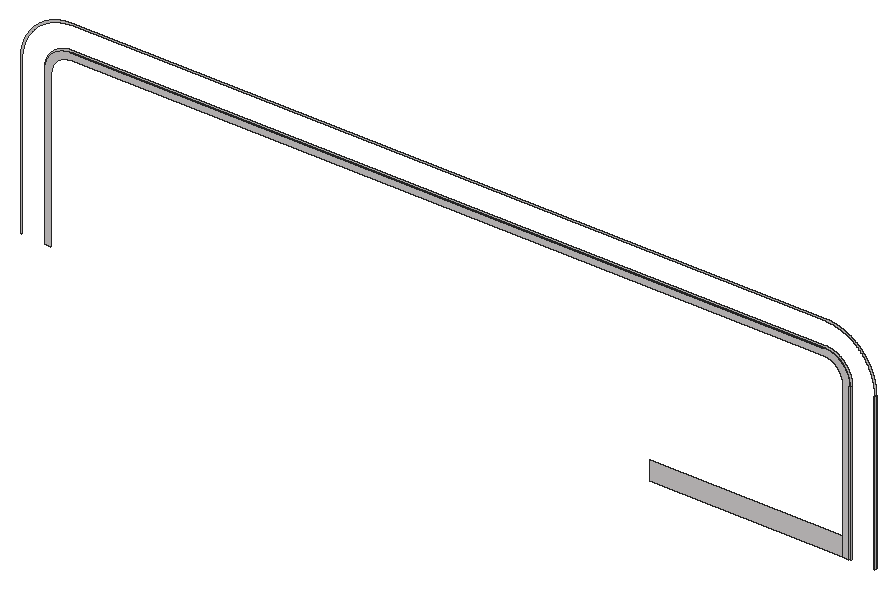
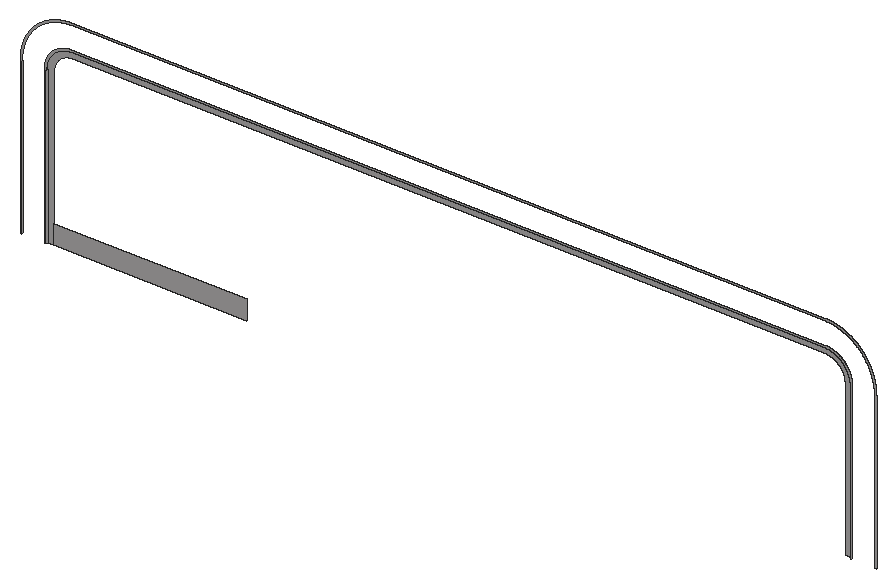
# SketchUp Ruby script. Lengths in inches.
U = 1.inch
M = Sketchup.active_model
def pt(a) = Geom::Point3d.new(a.map { |v| v * U })
def face(e, loops, mat)
  f = e.add_face(loops[0].map { |a| pt(a) })
  loops[1..].each { |l| e.add_face(l.map { |a| pt(a) }).erase! }
  f.material = f.back_material = mat if mat
  f
end
# faces: each face lists its corners as indices into pts; further lists are holes
def faces(e, pts, list, mat = nil) = list.each { |f| face(e, (f[0].is_a?(Array) ? f : [f]).map { |l| l.map { |i| pts[i] } }, mat) }
# xy, xz, yz: faces in a plane at the given z, y or x. An outline is a flat list of corners, or four numbers for a rectangle; further outlines are holes
def ring(l) = l.size == 4 ? [[l[0], l[1]], [l[2], l[1]], [l[2], l[3]], [l[0], l[3]]] : l.each_slice(2).to_a
def flat(e, list, mat, &to3) = list.each { |f| face(e, (f[0].is_a?(Array) ? f : [f]).map { |l| ring(l).map { |u, v| to3.(u, v) } }, mat) }
def xy(e, z, list, mat = nil) = flat(e, list, mat) { |x, y| [x, y, z] }
def xz(e, y, list, mat = nil) = flat(e, list, mat) { |x, z| [x, y, z] }
def yz(e, x, list, mat = nil) = flat(e, list, mat) { |y, z| [x, y, z] }
def lines(e, pts, list) = list.each { |a, b| e.add_line(pt(pts[a]), pt(pts[b])) }
# prism: a flat outline (further loops are holes) pulled along v
def prism(e, loops, v, mat = nil)
  f = face(e, loops, mat); d = Geom::Vector3d.new(v.map { |x| x * U })
  f.pushpull(f.normal.samedirection?(d) ? d.length : -d.length)
end
def box(e, o, s, mat = nil) = prism(e, [[o, [o[0] + s[0], o[1], o[2]], [o[0] + s[0], o[1] + s[1], o[2]], [o[0], o[1] + s[1], o[2]]]], [0, 0, s[2]], mat)
def at(x, y, z, deg = 0) = Geom::Transformation.translation(pt([x, y, z])) * Geom::Transformation.rotation(ORIGIN, Z_AXIS, deg.degrees)
def axes(o, x, y, z) = Geom::Transformation.new([*x, 0, *y, 0, *z, 0, *pt(o).to_a, 1])
def part(name) = M.definitions.add(name)
# library, detail: a bought-in or finely detailed component or shape, given as its bounding box
def library(name, o, s) = part(name).tap { |d| box(d.entities, o, s) }
def detail(e, o, s) = box(e.add_group.entities, o, s)
def put(e, d, t, mat = nil) = e.add_instance(d, t).tap { |i| i.material = mat if mat }
def group(e, t, mat = nil) = e.add_group.tap { |g| g.transformation = t; g.material = mat if mat }.entities
root = M.entities
M.materials.add("[Quartz Light Brown]").color = [215, 212, 212]
xz(root,38,[[20,-12,24,-12,24,84.28,24.01,84.375,24.01,84.57,24.02,84.66,24.02,84.75,24.03,84.85,24.04,84.94,24.04,85.04,24.05,85.13,24.0625,85.22,24.07,85.32,24.09,85.5,24.11,85.6,24.13,85.78,24.15,85.88,24.16,85.97,24.18,86.0625,24.2,86.16,24.21,86.25,24.25,86.43,24.27,86.53,24.35,86.89,24.38,86.98,24.4,87.08,24.43,87.17,24.45,87.26,24.48,87.35,24.5,87.4375,24.53,87.53,24.68,87.98,24.71,88.06,24.77,88.24,24.81,88.33,24.84,88.42,24.88,88.5,24.91,88.59,24.99,88.77,25.02,88.85,25.0625,88.9375,25.1,89.02,25.14,89.11,25.18,89.19,25.22,89.28,25.27,89.36,25.31,89.45,25.35,89.53,25.39,89.62,25.4375,89.7,25.48,89.78,25.53,89.86,25.58,89.95,25.67,90.11,25.72,90.1875,25.77,90.27,26.02,90.67,26.08,90.75,26.13,90.82,26.18,90.9,26.24,90.98,26.29,91.05,26.35,91.13,26.4,91.21,26.52,91.35,26.58,91.43,26.63,91.5,26.69,91.58,26.75,91.65,26.9375,91.86,27,91.9375,27.0625,92.01,27.1875,92.15,27.25,92.21,27.32,92.28,27.38,92.35,27.45,92.42,27.51,92.49,27.58,92.55,27.65,92.62,27.72,92.68,27.79,92.75,27.85,92.8125,27.99,92.9375,28.0625,93,28.14,93.0625,28.35,93.25,28.42,93.31,28.5,93.37,28.57,93.42,28.65,93.48,28.79,93.6,28.87,93.65,28.95,93.71,29.02,93.76,29.1,93.82,29.18,93.87,29.25,93.92,29.33,93.98,29.73,94.23,29.8125,94.28,29.89,94.33,30.05,94.42,30.14,94.47,30.22,94.52,30.3,94.5625,30.38,94.61,30.47,94.65,30.55,94.69,30.64,94.73,30.72,94.78,30.81,94.82,30.89,94.86,30.98,94.9,31.0625,94.9375,31.15,94.98,31.23,95.01,31.41,95.09,31.5,95.12,31.58,95.16,31.67,95.19,31.76,95.23,31.94,95.29,32.02,95.32,32.47,95.47,32.5625,95.5,32.65,95.52,32.74,95.55,32.83,95.57,32.92,95.6,33.02,95.62,33.11,95.65,33.47,95.73,33.57,95.75,33.75,95.79,33.84,95.8,33.9375,95.82,34.03,95.84,34.12,95.85,34.22,95.87,34.4,95.89,34.5,95.91,34.68,95.93,34.78,95.9375,34.87,95.95,34.96,95.96,35.06,95.96,35.15,95.97,35.25,95.98,35.34,95.98,35.43,95.99,35.625,95.99,35.72,96,504.28,96,504.375,95.99,504.57,95.99,504.66,95.98,504.75,95.98,504.85,95.97,504.94,95.96,505.04,95.96,505.13,95.95,505.22,95.9375,505.32,95.93,505.5,95.91,505.6,95.89,505.78,95.87,505.88,95.85,505.97,95.84,506.0625,95.82,506.16,95.8,506.25,95.79,506.43,95.75,506.53,95.73,506.89,95.65,506.98,95.62,507.08,95.6,507.17,95.57,507.26,95.55,507.35,95.52,507.4375,95.5,507.53,95.47,507.98,95.32,508.06,95.29,508.24,95.23,508.33,95.19,508.42,95.16,508.5,95.12,508.59,95.09,508.77,95.01,508.85,94.98,508.9375,94.9375,509.02,94.9,509.11,94.86,509.19,94.82,509.28,94.78,509.36,94.73,509.45,94.69,509.53,94.65,509.62,94.61,509.7,94.5625,509.78,94.52,509.86,94.47,509.95,94.42,510.11,94.33,510.1875,94.28,510.27,94.23,510.67,93.98,510.75,93.92,510.82,93.87,510.9,93.82,510.98,93.76,511.05,93.71,511.13,93.65,511.21,93.6,511.35,93.48,511.43,93.42,511.5,93.37,511.58,93.31,511.65,93.25,511.86,93.0625,511.9375,93,512.01,92.9375,512.15,92.8125,512.21,92.75,512.28,92.68,512.35,92.62,512.42,92.55,512.49,92.49,512.55,92.42,512.62,92.35,512.68,92.28,512.75,92.21,512.8125,92.15,512.9375,92.01,513,91.9375,513.0625,91.86,513.25,91.65,513.31,91.58,513.37,91.5,513.42,91.43,513.48,91.35,513.6,91.21,513.65,91.13,513.71,91.05,513.76,90.98,513.82,90.9,513.87,90.82,513.92,90.75,513.98,90.67,514.23,90.27,514.28,90.1875,514.33,90.11,514.42,89.95,514.47,89.86,514.52,89.78,514.5625,89.7,514.61,89.62,514.65,89.53,514.69,89.45,514.73,89.36,514.78,89.28,514.82,89.19,514.86,89.11,514.9,89.02,514.9375,88.9375,514.98,88.85,515.01,88.77,515.09,88.59,515.12,88.5,515.16,88.42,515.19,88.33,515.23,88.24,515.29,88.06,515.32,87.98,515.47,87.53,515.5,87.4375,515.52,87.35,515.55,87.26,515.57,87.17,515.6,87.08,515.62,86.98,515.65,86.89,515.73,86.53,515.75,86.43,515.79,86.25,515.8,86.16,515.82,86.0625,515.84,85.97,515.85,85.88,515.87,85.78,515.89,85.6,515.91,85.5,515.93,85.32,515.9375,85.22,515.95,85.13,515.96,85.04,515.96,84.94,515.97,84.85,515.98,84.75,515.98,84.66,515.99,84.57,515.99,84.375,516,84.28,516,-12,520,-12,520,84.375,519.99,84.5,519.99,84.63,519.98,84.75,519.98,84.88,519.97,85,519.95,85.26,519.94,85.38,519.93,85.51,519.92,85.63,519.9,85.76,519.89,85.88,519.875,86.01,519.86,86.13,519.84,86.25,519.82,86.38,519.8,86.5,519.72,87,519.69,87.12,519.67,87.24,519.64,87.37,519.61,87.49,519.59,87.61,519.56,87.74,519.47,88.1,519.43,88.22,519.4,88.34,519.36,88.46,519.33,88.58,519.29,88.7,519.26,88.82,519.22,88.94,519.18,89.0625,519.14,89.18,519.1,89.3,519.05,89.42,518.97,89.66,518.92,89.77,518.83,90.01,518.78,90.12,518.73,90.24,518.68,90.35,518.63,90.47,518.58,90.58,518.53,90.7,518.48,90.8125,518.42,90.93,518.37,91.04,518.3125,91.15,518.26,91.26,518.14,91.49,517.84,92.04,517.77,92.14,517.71,92.25,517.64,92.36,517.58,92.47,517.51,92.57,517.44,92.68,517.37,92.78,517.3,92.89,517.23,92.99,517.16,93.1,517.02,93.3,516.94,93.4,516.87,93.51,516.79,93.61,516.72,93.71,516.56,93.91,516.49,94,516.25,94.3,516.17,94.39,516.08,94.49,515.92,94.67,515.83,94.77,515.75,94.86,515.66,94.95,515.58,95.04,515.4,95.22,515.3125,95.3125,515.22,95.4,515.04,95.58,514.95,95.66,514.86,95.75,514.77,95.83,514.67,95.92,514.49,96.08,514.39,96.17,514.3,96.25,514,96.49,513.91,96.56,513.71,96.72,513.61,96.79,513.51,96.87,513.4,96.94,513.3,97.02,513.1,97.16,512.99,97.23,512.89,97.3,512.78,97.37,512.68,97.44,512.57,97.51,512.47,97.58,512.36,97.64,512.25,97.71,512.14,97.77,512.04,97.84,511.49,98.14,511.26,98.26,511.15,98.3125,511.04,98.37,510.93,98.42,510.8125,98.48,510.7,98.53,510.58,98.58,510.47,98.63,510.35,98.68,510.24,98.73,510.12,98.78,510.01,98.83,509.77,98.92,509.66,98.97,509.42,99.05,509.3,99.1,509.18,99.14,509.0625,99.18,508.94,99.22,508.82,99.26,508.7,99.29,508.58,99.33,508.46,99.36,508.34,99.4,508.22,99.43,508.1,99.47,507.74,99.56,507.61,99.59,507.49,99.61,507.37,99.64,507.24,99.67,507.12,99.69,507,99.72,506.5,99.8,506.38,99.82,506.25,99.84,506.13,99.86,506.01,99.875,505.88,99.89,505.76,99.9,505.63,99.92,505.51,99.93,505.38,99.94,505.26,99.95,505,99.97,504.88,99.98,504.75,99.98,504.63,99.99,504.5,99.99,504.375,100,35.625,100,35.5,99.99,35.37,99.99,35.25,99.98,35.12,99.98,35,99.97,34.74,99.95,34.62,99.94,34.49,99.93,34.37,99.92,34.24,99.9,34.12,99.89,33.99,99.875,33.87,99.86,33.75,99.84,33.62,99.82,33.5,99.8,33,99.72,32.88,99.69,32.76,99.67,32.63,99.64,32.51,99.61,32.39,99.59,32.26,99.56,31.9,99.47,31.78,99.43,31.66,99.4,31.54,99.36,31.42,99.33,31.3,99.29,31.18,99.26,31.06,99.22,30.9375,99.18,30.82,99.14,30.7,99.1,30.58,99.05,30.34,98.97,30.23,98.92,29.99,98.83,29.88,98.78,29.76,98.73,29.65,98.68,29.53,98.63,29.42,98.58,29.3,98.53,29.1875,98.48,29.07,98.42,28.96,98.37,28.85,98.3125,28.74,98.26,28.51,98.14,27.96,97.84,27.86,97.77,27.75,97.71,27.64,97.64,27.53,97.58,27.43,97.51,27.32,97.44,27.22,97.37,27.11,97.3,27.01,97.23,26.9,97.16,26.7,97.02,26.6,96.94,26.49,96.87,26.39,96.79,26.29,96.72,26.09,96.56,26,96.49,25.7,96.25,25.61,96.17,25.51,96.08,25.33,95.92,25.23,95.83,25.14,95.75,25.05,95.66,24.96,95.58,24.78,95.4,24.6875,95.3125,24.6,95.22,24.42,95.04,24.34,94.95,24.25,94.86,24.17,94.77,24.08,94.67,23.92,94.49,23.83,94.39,23.75,94.3,23.51,94,23.44,93.91,23.28,93.71,23.21,93.61,23.13,93.51,23.06,93.4,22.98,93.3,22.84,93.1,22.77,92.99,22.7,92.89,22.63,92.78,22.56,92.68,22.49,92.57,22.42,92.47,22.36,92.36,22.29,92.25,22.23,92.14,22.16,92.04,21.86,91.49,21.74,91.26,21.6875,91.15,21.63,91.04,21.58,90.93,21.52,90.8125,21.47,90.7,21.42,90.58,21.37,90.47,21.32,90.35,21.27,90.24,21.22,90.12,21.17,90.01,21.08,89.77,21.03,89.66,20.95,89.42,20.9,89.3,20.86,89.18,20.82,89.0625,20.78,88.94,20.74,88.82,20.71,88.7,20.67,88.58,20.64,88.46,20.6,88.34,20.57,88.22,20.53,88.1,20.44,87.74,20.41,87.61,20.39,87.49,20.36,87.37,20.33,87.24,20.31,87.12,20.28,87,20.2,86.5,20.18,86.38,20.16,86.25,20.14,86.13,20.125,86.01,20.11,85.88,20.1,85.76,20.08,85.63,20.07,85.51,20.06,85.38,20.05,85.26,20.03,85,20.02,84.88,20.02,84.75,20.01,84.63,20.01,84.5,20,84.375],[396,-12,516,0]],"[Quartz Light Brown]")
xz(root,39,[[4,-12,5,-12,5,84.49,5.02,84.97,5.02,85.22,5.03,85.46,5.05,85.7,5.0625,85.95,5.08,86.1875,5.1,86.43,5.12,86.67,5.14,86.92,5.16,87.16,5.1875,87.4,5.21,87.64,5.24,87.89,5.28,88.125,5.31,88.37,5.34,88.61,5.5,89.57,5.6,90.05,5.64,90.29,5.69,90.52,5.75,90.76,5.8,91,5.86,91.24,5.91,91.47,5.97,91.71,6.04,91.94,6.1,92.18,6.16,92.41,6.23,92.65,6.3,92.88,6.37,93.12,6.44,93.35,6.52,93.58,6.59,93.8125,6.67,94.04,6.83,94.5,6.92,94.73,7,94.96,7.09,95.19,7.18,95.41,7.27,95.64,7.36,95.86,7.45,96.09,7.55,96.3125,7.65,96.53,7.75,96.76,8.05,97.42,8.27,97.86,8.38,98.07,8.6,98.51,8.72,98.72,8.83,98.93,8.95,99.15,9.19,99.57,9.32,99.78,9.44,99.99,9.57,100.2,9.7,100.4,9.96,100.82,10.22,101.22,10.36,101.42,10.64,101.83,10.78,102.02,10.92,102.22,11.0625,102.42,11.21,102.61,11.36,102.81,12.11,103.76,12.27,103.95,12.43,104.13,12.59,104.32,13.07,104.86,13.24,105.04,13.4,105.22,13.57,105.4,13.74,105.57,13.91,105.75,14.25,106.09,14.43,106.26,14.6,106.43,14.78,106.6,14.96,106.76,15.14,106.93,15.68,107.41,15.87,107.57,16.05,107.73,16.24,107.89,17.19,108.64,17.39,108.79,17.58,108.9375,17.78,109.08,17.98,109.22,18.17,109.36,18.58,109.64,18.78,109.78,19.18,110.04,19.6,110.3,19.8,110.43,20.01,110.56,20.22,110.68,20.43,110.81,20.85,111.05,21.07,111.17,21.28,111.28,21.49,111.4,21.93,111.62,22.14,111.73,22.58,111.95,23.24,112.25,23.47,112.35,23.6875,112.45,23.91,112.55,24.14,112.64,24.36,112.73,24.59,112.82,24.81,112.91,25.04,113,25.27,113.08,25.5,113.17,25.96,113.33,26.1875,113.41,26.42,113.48,26.65,113.56,26.88,113.63,27.12,113.7,27.35,113.77,27.59,113.84,27.82,113.9,28.06,113.96,28.29,114.03,28.53,114.09,28.76,114.14,29,114.2,29.24,114.25,29.48,114.31,29.71,114.36,29.95,114.4,30.43,114.5,31.39,114.66,31.63,114.69,31.875,114.72,32.11,114.76,32.36,114.79,32.6,114.8125,32.84,114.84,33.08,114.86,33.33,114.88,33.57,114.9,33.8125,114.92,34.05,114.9375,34.3,114.95,34.54,114.97,34.78,114.98,35.03,114.98,35.51,115,504.49,115,504.97,114.98,505.22,114.98,505.46,114.97,505.7,114.95,505.95,114.9375,506.1875,114.92,506.43,114.9,506.67,114.88,506.92,114.86,507.16,114.84,507.4,114.8125,507.64,114.79,507.89,114.76,508.125,114.72,508.37,114.69,508.61,114.66,509.57,114.5,510.05,114.4,510.29,114.36,510.52,114.31,510.76,114.25,511,114.2,511.24,114.14,511.47,114.09,511.71,114.03,511.94,113.96,512.18,113.9,512.41,113.84,512.65,113.77,512.88,113.7,513.12,113.63,513.35,113.56,513.58,113.48,513.8125,113.41,514.04,113.33,514.5,113.17,514.73,113.08,514.96,113,515.19,112.91,515.41,112.82,515.64,112.73,515.86,112.64,516.09,112.55,516.3125,112.45,516.53,112.35,516.76,112.25,517.42,111.95,517.86,111.73,518.07,111.62,518.51,111.4,518.72,111.28,518.93,111.17,519.15,111.05,519.57,110.81,519.78,110.68,519.99,110.56,520.2,110.43,520.4,110.3,520.82,110.04,521.22,109.78,521.42,109.64,521.83,109.36,522.02,109.22,522.22,109.08,522.42,108.9375,522.61,108.79,522.81,108.64,523.76,107.89,523.95,107.73,524.13,107.57,524.32,107.41,524.86,106.93,525.04,106.76,525.22,106.6,525.4,106.43,525.57,106.26,525.75,106.09,526.09,105.75,526.26,105.57,526.43,105.4,526.6,105.22,526.76,105.04,526.93,104.86,527.41,104.32,527.57,104.13,527.73,103.95,527.89,103.76,528.64,102.81,528.79,102.61,528.9375,102.42,529.08,102.22,529.22,102.02,529.36,101.83,529.64,101.42,529.78,101.22,530.04,100.82,530.3,100.4,530.43,100.2,530.56,99.99,530.68,99.78,530.81,99.57,531.05,99.15,531.17,98.93,531.28,98.72,531.4,98.51,531.62,98.07,531.73,97.86,531.95,97.42,532.25,96.76,532.35,96.53,532.45,96.3125,532.55,96.09,532.64,95.86,532.73,95.64,532.82,95.41,532.91,95.19,533,94.96,533.08,94.73,533.17,94.5,533.33,94.04,533.41,93.8125,533.48,93.58,533.56,93.35,533.63,93.12,533.7,92.88,533.77,92.65,533.84,92.41,533.9,92.18,533.96,91.94,534.03,91.71,534.09,91.47,534.14,91.24,534.2,91,534.25,90.76,534.31,90.52,534.36,90.29,534.4,90.05,534.5,89.57,534.66,88.61,534.69,88.37,534.72,88.125,534.76,87.89,534.79,87.64,534.8125,87.4,534.84,87.16,534.86,86.92,534.88,86.67,534.9,86.43,534.92,86.1875,534.9375,85.95,534.95,85.7,534.97,85.46,534.98,85.22,534.98,84.97,535,84.49,535,-12,536,-12,536,84.5,535.99,84.75,535.98,85.01,535.98,85.26,535.96,85.51,535.95,85.76,535.9375,86.01,535.92,86.26,535.86,87.01,535.83,87.26,535.81,87.51,535.72,88.26,535.64,88.76,535.61,89.01,535.57,89.25,535.52,89.5,535.48,89.75,535.43,90,535.39,90.24,535.34,90.49,535.28,90.74,535.23,90.98,535.17,91.23,535.12,91.47,535.06,91.71,534.99,91.96,534.87,92.44,534.8,92.6875,534.73,92.93,534.59,93.41,534.43,93.89,534.36,94.13,534.27,94.37,534.19,94.6,534.11,94.84,534.02,95.08,533.93,95.3125,533.84,95.55,533.66,96.01,533.5625,96.25,533.47,96.48,533.37,96.71,533.27,96.9375,533.16,97.17,533.0625,97.4,532.95,97.625,532.85,97.85,532.74,98.08,532.625,98.3,532.4,98.75,532.28,98.97,532.16,99.2,531.92,99.64,531.8,99.85,531.41,100.51,531.15,100.93,531.02,101.15,530.88,101.36,530.75,101.57,530.47,101.99,530.32,102.19,530.04,102.61,529.59,103.21,529.4375,103.41,529.28,103.61,529.13,103.8125,528.97,104.01,528.82,104.2,528.66,104.4,528.5,104.59,528.33,104.78,528.17,104.97,528,105.16,527.84,105.35,527.67,105.54,527.5,105.72,527.33,105.91,527.15,106.09,526.98,106.27,526.8,106.45,526.63,106.63,526.45,106.8,526.27,106.98,526.09,107.15,525.91,107.33,525.72,107.5,525.54,107.67,525.35,107.84,525.16,108,524.97,108.17,524.78,108.33,524.59,108.5,524.4,108.66,524.2,108.82,524.01,108.97,523.8125,109.13,523.61,109.28,523.41,109.4375,523.21,109.59,522.61,110.04,522.19,110.32,521.99,110.47,521.57,110.75,521.36,110.88,521.15,111.02,520.93,111.15,520.51,111.41,519.85,111.8,519.64,111.92,519.2,112.16,518.97,112.28,518.75,112.4,518.3,112.625,518.08,112.74,517.85,112.85,517.625,112.95,517.4,113.0625,517.17,113.16,516.9375,113.27,516.71,113.37,516.48,113.47,516.25,113.5625,516.01,113.66,515.55,113.84,515.3125,113.93,515.08,114.02,514.84,114.11,514.6,114.19,514.37,114.27,514.13,114.36,513.89,114.43,513.41,114.59,512.93,114.73,512.6875,114.8,512.44,114.87,511.96,114.99,511.71,115.06,511.47,115.12,511.23,115.17,510.98,115.23,510.74,115.28,510.49,115.34,510.24,115.39,510,115.43,509.75,115.48,509.5,115.52,509.25,115.57,509.01,115.61,508.76,115.64,508.26,115.72,507.51,115.81,507.26,115.83,507.01,115.86,506.26,115.92,506.01,115.9375,505.76,115.95,505.51,115.96,505.26,115.98,505.01,115.98,504.75,115.99,504.5,116,35.5,116,35.25,115.99,34.99,115.98,34.74,115.98,34.49,115.96,34.24,115.95,33.99,115.9375,33.74,115.92,32.99,115.86,32.74,115.83,32.49,115.81,31.74,115.72,31.24,115.64,30.99,115.61,30.75,115.57,30.5,115.52,30.25,115.48,30,115.43,29.76,115.39,29.51,115.34,29.26,115.28,29.02,115.23,28.77,115.17,28.53,115.12,28.29,115.06,28.04,114.99,27.56,114.87,27.3125,114.8,27.07,114.73,26.59,114.59,26.11,114.43,25.87,114.36,25.63,114.27,25.4,114.19,25.16,114.11,24.92,114.02,24.6875,113.93,24.45,113.84,23.99,113.66,23.75,113.5625,23.52,113.47,23.29,113.37,23.0625,113.27,22.83,113.16,22.6,113.0625,22.375,112.95,22.15,112.85,21.92,112.74,21.7,112.625,21.25,112.4,21.03,112.28,20.8,112.16,20.36,111.92,20.15,111.8,19.49,111.41,19.07,111.15,18.85,111.02,18.64,110.88,18.43,110.75,18.01,110.47,17.81,110.32,17.39,110.04,16.79,109.59,16.59,109.4375,16.39,109.28,16.1875,109.13,15.99,108.97,15.8,108.82,15.6,108.66,15.41,108.5,15.22,108.33,15.03,108.17,14.84,108,14.65,107.84,14.46,107.67,14.28,107.5,14.09,107.33,13.91,107.15,13.73,106.98,13.55,106.8,13.37,106.63,13.2,106.45,13.02,106.27,12.85,106.09,12.67,105.91,12.5,105.72,12.33,105.54,12.16,105.35,12,105.16,11.83,104.97,11.67,104.78,11.5,104.59,11.34,104.4,11.18,104.2,11.03,104.01,10.87,103.8125,10.72,103.61,10.5625,103.41,10.41,103.21,9.96,102.61,9.68,102.19,9.53,101.99,9.25,101.57,9.12,101.36,8.98,101.15,8.85,100.93,8.59,100.51,8.2,99.85,8.08,99.64,7.84,99.2,7.72,98.97,7.6,98.75,7.375,98.3,7.26,98.08,7.15,97.85,7.05,97.625,6.9375,97.4,6.84,97.17,6.73,96.9375,6.63,96.71,6.53,96.48,6.4375,96.25,6.34,96.01,6.16,95.55,6.07,95.3125,5.98,95.08,5.89,94.84,5.81,94.6,5.73,94.37,5.64,94.13,5.57,93.89,5.41,93.41,5.27,92.93,5.2,92.6875,5.13,92.44,5.01,91.96,4.94,91.71,4.88,91.47,4.83,91.23,4.77,90.98,4.72,90.74,4.66,90.49,4.61,90.24,4.57,90,4.52,89.75,4.48,89.5,4.43,89.25,4.39,89.01,4.36,88.76,4.28,88.26,4.19,87.51,4.17,87.26,4.14,87.01,4.08,86.26,4.0625,86.01,4.05,85.76,4.04,85.51,4.02,85.26,4.02,85.01,4.01,84.75,4,84.5],[19,-12,20,-12,20,84.375,20.01,84.5,20.01,84.63,20.02,84.75,20.02,84.88,20.03,85,20.05,85.26,20.06,85.38,20.07,85.51,20.08,85.63,20.1,85.76,20.11,85.88,20.125,86.01,20.14,86.13,20.16,86.25,20.18,86.38,20.2,86.5,20.28,87,20.31,87.12,20.33,87.24,20.36,87.37,20.39,87.49,20.41,87.61,20.44,87.74,20.53,88.1,20.57,88.22,20.6,88.34,20.64,88.46,20.67,88.58,20.71,88.7,20.74,88.82,20.78,88.94,20.82,89.0625,20.86,89.18,20.9,89.3,20.95,89.42,21.03,89.66,21.08,89.77,21.17,90.01,21.22,90.12,21.27,90.24,21.32,90.35,21.37,90.47,21.42,90.58,21.47,90.7,21.52,90.8125,21.58,90.93,21.63,91.04,21.6875,91.15,21.74,91.26,21.86,91.49,22.16,92.04,22.23,92.14,22.29,92.25,22.36,92.36,22.42,92.47,22.49,92.57,22.56,92.68,22.63,92.78,22.7,92.89,22.77,92.99,22.84,93.1,22.98,93.3,23.06,93.4,23.13,93.51,23.21,93.61,23.28,93.71,23.44,93.91,23.51,94,23.75,94.3,23.83,94.39,23.92,94.49,24.08,94.67,24.17,94.77,24.25,94.86,24.34,94.95,24.42,95.04,24.6,95.22,24.6875,95.3125,24.78,95.4,24.96,95.58,25.05,95.66,25.14,95.75,25.23,95.83,25.33,95.92,25.51,96.08,25.61,96.17,25.7,96.25,26,96.49,26.09,96.56,26.29,96.72,26.39,96.79,26.49,96.87,26.6,96.94,26.7,97.02,26.9,97.16,27.01,97.23,27.11,97.3,27.22,97.37,27.32,97.44,27.43,97.51,27.53,97.58,27.64,97.64,27.75,97.71,27.86,97.77,27.96,97.84,28.51,98.14,28.74,98.26,28.85,98.3125,28.96,98.37,29.07,98.42,29.1875,98.48,29.3,98.53,29.42,98.58,29.53,98.63,29.65,98.68,29.76,98.73,29.88,98.78,29.99,98.83,30.23,98.92,30.34,98.97,30.58,99.05,30.7,99.1,30.82,99.14,30.9375,99.18,31.06,99.22,31.18,99.26,31.3,99.29,31.42,99.33,31.54,99.36,31.66,99.4,31.78,99.43,31.9,99.47,32.26,99.56,32.39,99.59,32.51,99.61,32.63,99.64,32.76,99.67,32.88,99.69,33,99.72,33.5,99.8,33.62,99.82,33.75,99.84,33.87,99.86,33.99,99.875,34.12,99.89,34.24,99.9,34.37,99.92,34.49,99.93,34.62,99.94,34.74,99.95,35,99.97,35.12,99.98,35.25,99.98,35.37,99.99,35.5,99.99,35.625,100,504.375,100,504.5,99.99,504.63,99.99,504.75,99.98,504.88,99.98,505,99.97,505.26,99.95,505.38,99.94,505.51,99.93,505.63,99.92,505.76,99.9,505.88,99.89,506.01,99.875,506.13,99.86,506.25,99.84,506.38,99.82,506.5,99.8,507,99.72,507.12,99.69,507.24,99.67,507.37,99.64,507.49,99.61,507.61,99.59,507.74,99.56,508.1,99.47,508.22,99.43,508.34,99.4,508.46,99.36,508.58,99.33,508.7,99.29,508.82,99.26,508.94,99.22,509.0625,99.18,509.18,99.14,509.3,99.1,509.42,99.05,509.66,98.97,509.77,98.92,510.01,98.83,510.12,98.78,510.24,98.73,510.35,98.68,510.47,98.63,510.58,98.58,510.7,98.53,510.8125,98.48,510.93,98.42,511.04,98.37,511.15,98.3125,511.26,98.26,511.49,98.14,512.04,97.84,512.14,97.77,512.25,97.71,512.36,97.64,512.47,97.58,512.57,97.51,512.68,97.44,512.78,97.37,512.89,97.3,512.99,97.23,513.1,97.16,513.3,97.02,513.4,96.94,513.51,96.87,513.61,96.79,513.71,96.72,513.91,96.56,514,96.49,514.3,96.25,514.39,96.17,514.49,96.08,514.67,95.92,514.77,95.83,514.86,95.75,514.95,95.66,515.04,95.58,515.22,95.4,515.3125,95.3125,515.4,95.22,515.58,95.04,515.66,94.95,515.75,94.86,515.83,94.77,515.92,94.67,516.08,94.49,516.17,94.39,516.25,94.3,516.49,94,516.56,93.91,516.72,93.71,516.79,93.61,516.87,93.51,516.94,93.4,517.02,93.3,517.16,93.1,517.23,92.99,517.3,92.89,517.37,92.78,517.44,92.68,517.51,92.57,517.58,92.47,517.64,92.36,517.71,92.25,517.77,92.14,517.84,92.04,518.14,91.49,518.26,91.26,518.3125,91.15,518.37,91.04,518.42,90.93,518.48,90.8125,518.53,90.7,518.58,90.58,518.63,90.47,518.68,90.35,518.73,90.24,518.78,90.12,518.83,90.01,518.92,89.77,518.97,89.66,519.05,89.42,519.1,89.3,519.14,89.18,519.18,89.0625,519.22,88.94,519.26,88.82,519.29,88.7,519.33,88.58,519.36,88.46,519.4,88.34,519.43,88.22,519.47,88.1,519.56,87.74,519.59,87.61,519.61,87.49,519.64,87.37,519.67,87.24,519.69,87.12,519.72,87,519.8,86.5,519.82,86.38,519.84,86.25,519.86,86.13,519.875,86.01,519.89,85.88,519.9,85.76,519.92,85.63,519.93,85.51,519.94,85.38,519.95,85.26,519.97,85,519.98,84.88,519.98,84.75,519.99,84.63,519.99,84.5,520,84.375,520,-12,521,-12,521,84.4,520.99,84.53,520.99,84.67,520.97,84.93,520.97,85.07,520.95,85.33,520.9375,85.47,520.92,85.6,520.91,85.73,520.9,85.87,520.88,86,520.87,86.13,520.85,86.26,520.83,86.4,520.8125,86.53,520.79,86.66,520.75,86.92,520.72,87.05,520.7,87.19,520.67,87.32,520.65,87.45,520.59,87.71,520.5625,87.84,520.53,87.97,520.47,88.23,520.43,88.36,520.4,88.49,520.36,88.61,520.32,88.74,520.29,88.87,520.25,89,520.17,89.25,520.08,89.51,520.04,89.63,519.99,89.76,519.95,89.88,519.9,90.01,519.85,90.13,519.81,90.26,519.76,90.38,519.71,90.51,519.65,90.63,519.6,90.75,519.55,90.875,519.49,91,519.4375,91.12,519.38,91.24,519.32,91.36,519.27,91.48,519.09,91.84,519.02,91.95,518.9,92.19,518.83,92.31,518.77,92.42,518.7,92.54,518.63,92.65,518.5625,92.77,518.49,92.88,518.42,93,518.21,93.33,518.13,93.44,518.06,93.56,517.98,93.67,517.91,93.78,517.83,93.88,517.59,94.21,517.51,94.3125,517.43,94.42,517.35,94.52,517.27,94.63,517.18,94.73,517.1,94.84,517.01,94.9375,516.93,95.04,516.39,95.64,516.3,95.73,516.21,95.83,515.83,96.21,515.73,96.3,515.64,96.39,515.04,96.93,514.9375,97.01,514.84,97.1,514.73,97.18,514.63,97.27,514.52,97.35,514.42,97.43,514.3125,97.51,514.21,97.59,513.88,97.83,513.78,97.91,513.67,97.98,513.56,98.06,513.44,98.13,513.33,98.21,513,98.42,512.88,98.49,512.77,98.5625,512.65,98.63,512.54,98.7,512.42,98.77,512.31,98.83,512.19,98.9,511.95,99.02,511.84,99.09,511.48,99.27,511.36,99.32,511.24,99.38,511.12,99.4375,511,99.49,510.875,99.55,510.75,99.6,510.63,99.65,510.51,99.71,510.38,99.76,510.26,99.81,510.13,99.85,510.01,99.9,509.88,99.95,509.76,99.99,509.63,100.04,509.51,100.08,509.25,100.17,509,100.25,508.87,100.29,508.74,100.32,508.61,100.36,508.49,100.4,508.36,100.43,508.23,100.47,507.97,100.53,507.84,100.5625,507.71,100.59,507.45,100.65,507.32,100.67,507.19,100.7,507.05,100.72,506.92,100.75,506.66,100.79,506.53,100.8125,506.4,100.83,506.26,100.85,506.13,100.87,506,100.88,505.87,100.9,505.73,100.91,505.6,100.92,505.47,100.9375,505.33,100.95,505.07,100.97,504.93,100.97,504.67,100.99,504.53,100.99,504.4,101,35.6,101,35.47,100.99,35.33,100.99,35.07,100.97,34.93,100.97,34.67,100.95,34.53,100.9375,34.4,100.92,34.27,100.91,34.13,100.9,34,100.88,33.87,100.87,33.74,100.85,33.6,100.83,33.47,100.8125,33.34,100.79,33.08,100.75,32.95,100.72,32.81,100.7,32.68,100.67,32.55,100.65,32.29,100.59,32.16,100.5625,32.03,100.53,31.77,100.47,31.64,100.43,31.51,100.4,31.39,100.36,31.26,100.32,31.13,100.29,31,100.25,30.75,100.17,30.49,100.08,30.37,100.04,30.24,99.99,30.12,99.95,29.99,99.9,29.87,99.85,29.74,99.81,29.62,99.76,29.49,99.71,29.37,99.65,29.25,99.6,29.125,99.55,29,99.49,28.88,99.4375,28.76,99.38,28.64,99.32,28.52,99.27,28.16,99.09,28.05,99.02,27.81,98.9,27.69,98.83,27.58,98.77,27.46,98.7,27.35,98.63,27.23,98.5625,27.12,98.49,27,98.42,26.67,98.21,26.56,98.13,26.44,98.06,26.33,97.98,26.22,97.91,26.12,97.83,25.79,97.59,25.6875,97.51,25.58,97.43,25.48,97.35,25.37,97.27,25.27,97.18,25.16,97.1,25.0625,97.01,24.96,96.93,24.36,96.39,24.27,96.3,24.17,96.21,23.79,95.83,23.7,95.73,23.61,95.64,23.07,95.04,22.99,94.9375,22.9,94.84,22.82,94.73,22.73,94.63,22.65,94.52,22.57,94.42,22.49,94.3125,22.41,94.21,22.17,93.88,22.09,93.78,22.02,93.67,21.94,93.56,21.87,93.44,21.79,93.33,21.58,93,21.51,92.88,21.4375,92.77,21.37,92.65,21.3,92.54,21.23,92.42,21.17,92.31,21.1,92.19,20.98,91.95,20.91,91.84,20.73,91.48,20.68,91.36,20.62,91.24,20.5625,91.12,20.51,91,20.45,90.875,20.4,90.75,20.35,90.63,20.29,90.51,20.24,90.38,20.19,90.26,20.15,90.13,20.1,90.01,20.05,89.88,20.01,89.76,19.96,89.63,19.92,89.51,19.83,89.25,19.75,89,19.71,88.87,19.68,88.74,19.64,88.61,19.6,88.49,19.57,88.36,19.53,88.23,19.47,87.97,19.4375,87.84,19.41,87.71,19.35,87.45,19.33,87.32,19.3,87.19,19.28,87.05,19.25,86.92,19.21,86.66,19.1875,86.53,19.17,86.4,19.15,86.26,19.13,86.13,19.12,86,19.1,85.87,19.09,85.73,19.08,85.6,19.0625,85.47,19.05,85.33,19.03,85.07,19.03,84.93,19.01,84.67,19.01,84.53,19,84.4]],"[Quartz Light Brown]")
yz(root,520,[[38,-12,39,83.96]],"[Quartz Light Brown]")
yz(root,521,[[38,-12,39,83.96]],"[Quartz Light Brown]")
yz(root,535,[[38,-12,39,83.99]],"[Quartz Light Brown]")
yz(root,536,[[38,-12,39,83.99]],"[Quartz Light Brown]")
